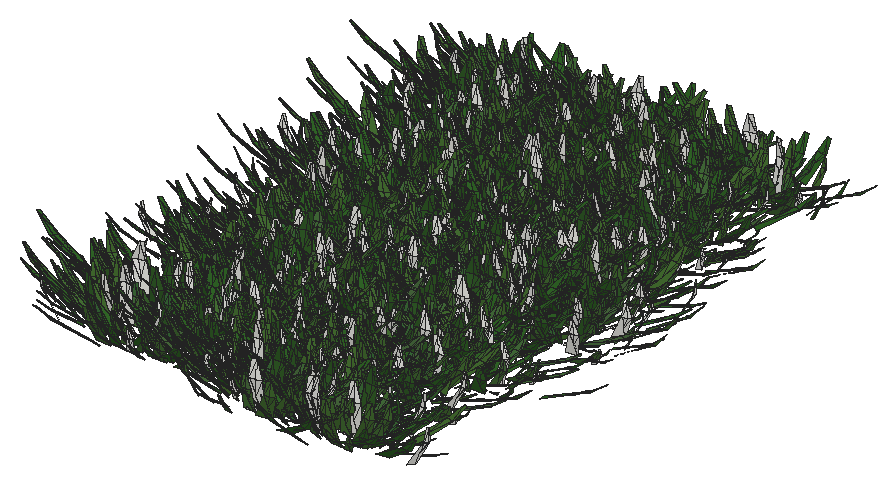
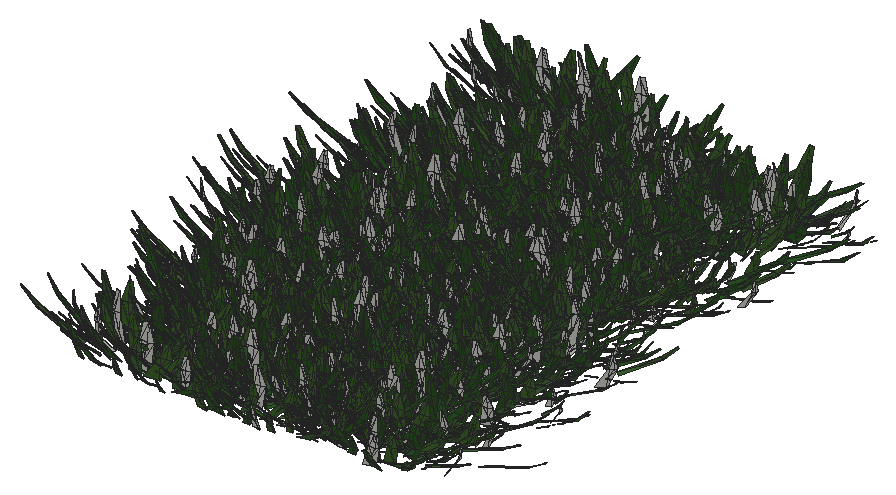
# SketchUp Ruby script. Lengths in inches.
U = 1.inch
M = Sketchup.active_model
def pt(a) = Geom::Point3d.new(a.map { |v| v * U })
def face(e, loops, mat)
  f = e.add_face(loops[0].map { |a| pt(a) })
  loops[1..].each { |l| e.add_face(l.map { |a| pt(a) }).erase! }
  f.material = f.back_material = mat if mat
  f
end
# faces: each face lists its corners as indices into pts; further lists are holes
def faces(e, pts, list, mat = nil) = list.each { |f| face(e, (f[0].is_a?(Array) ? f : [f]).map { |l| l.map { |i| pts[i] } }, mat) }
# xy, xz, yz: faces in a plane at the given z, y or x. An outline is a flat list of corners, or four numbers for a rectangle; further outlines are holes
def ring(l) = l.size == 4 ? [[l[0], l[1]], [l[2], l[1]], [l[2], l[3]], [l[0], l[3]]] : l.each_slice(2).to_a
def flat(e, list, mat, &to3) = list.each { |f| face(e, (f[0].is_a?(Array) ? f : [f]).map { |l| ring(l).map { |u, v| to3.(u, v) } }, mat) }
def xy(e, z, list, mat = nil) = flat(e, list, mat) { |x, y| [x, y, z] }
def xz(e, y, list, mat = nil) = flat(e, list, mat) { |x, z| [x, y, z] }
def yz(e, x, list, mat = nil) = flat(e, list, mat) { |y, z| [x, y, z] }
def lines(e, pts, list) = list.each { |a, b| e.add_line(pt(pts[a]), pt(pts[b])) }
# prism: a flat outline (further loops are holes) pulled along v
def prism(e, loops, v, mat = nil)
  f = face(e, loops, mat); d = Geom::Vector3d.new(v.map { |x| x * U })
  f.pushpull(f.normal.samedirection?(d) ? d.length : -d.length)
end
def box(e, o, s, mat = nil) = prism(e, [[o, [o[0] + s[0], o[1], o[2]], [o[0] + s[0], o[1] + s[1], o[2]], [o[0], o[1] + s[1], o[2]]]], [0, 0, s[2]], mat)
def at(x, y, z, deg = 0) = Geom::Transformation.translation(pt([x, y, z])) * Geom::Transformation.rotation(ORIGIN, Z_AXIS, deg.degrees)
def axes(o, x, y, z) = Geom::Transformation.new([*x, 0, *y, 0, *z, 0, *pt(o).to_a, 1])
def part(name) = M.definitions.add(name)
# library, detail: a bought-in or finely detailed component or shape, given as its bounding box
def library(name, o, s) = part(name).tap { |d| box(d.entities, o, s) }
def detail(e, o, s) = box(e.add_group.entities, o, s)
def put(e, d, t, mat = nil) = e.add_instance(d, t).tap { |i| i.material = mat if mat }
def group(e, t, mat = nil) = e.add_group.tap { |g| g.transformation = t; g.material = mat if mat }.entities
root = M.entities
M.materials.add("Material82").color = [68, 110, 58]
M.materials.add("Material83").color = [48, 90, 38]
M.materials.add("Material84").color = [68, 110, 48]
M.materials.add("Material85").color = [48, 90, 48]
M.materials.add("Material86").color = [58, 110, 58]
M.materials.add("Material87").color = [58, 90, 38]
M.materials.add("Material88").color = [68, 100, 58]
M.materials.add("Material89").color = [48, 100, 38]
c1 = part("grass00")
p = [[-0.6875,0.15,0],[-0.56,0.08,5.52],[-0.04,0.03,2.76],[0.48,-0.02,0],[0.35,-0.02,5.52],[-0.1,-0.14,5.52],
  [-0.12,0.65,8.37],[-0.42,0.65,8.37]]
faces(c1.entities,p,[[0,1,2,3],[3,2,4],[1,5,2],[5,4,2],[1,6,5],[4,5,6],[7,6,1]])
c2 = part("Group16\#1")
put(c2.entities,c1,axes([1.44,-0.61,-0.01],[0.05352,0.12609,0],[-0.10704,0.04543,0.07239],[0.06664,-0.02828,0.11628]),"Material85")
put(c2.entities,c1,axes([0.76,-0.15,-0.01],[0.04676,0.24062,0],[-0.23162,0.04501,0.06642],[0.0652,-0.01267,0.23595]),"Material82")
put(c2.entities,c1,axes([0.79,0.01,-0.01],[-0.00606,0.34651,0],[-0.34381,-0.00602,0.0432],[0.04319,0.00076,0.34386]))
put(c2.entities,c1,axes([1,0.23,-0.01],[-0.07192,0.31144,0],[-0.28722,-0.06632,0.1236],[0.12043,0.02781,0.29478]),"Material84")
put(c2.entities,c1,axes([1.66,0.77,-0.01],[-0.13828,0.29651,0],[-0.21551,-0.1005,0.22471],[0.20365,0.09498,0.23779]),"Material89")
put(c2.entities,c1,axes([0.6875,0.52,-0.01],[-0.18126,0.24051,0],[-0.22746,-0.17142,0.09788],[0.07817,0.05891,0.28481]),"Material84")
put(c2.entities,c1,axes([0.68,0.78,-0.01],[-0.215,0.18688,0],[-0.12385,-0.14248,0.21334],[0.13995,0.16101,0.18878]),"Material82")
put(c2.entities,c1,axes([0.56,1,-0.01],[-0.13756,0.07624,0],[-0.06159,-0.11112,0.0927],[0.04494,0.08108,0.12705]),"Material84")
put(c2.entities,c1,axes([0.2,0.64,-0.01],[-0.23729,0.07254,0],[-0.05711,-0.18681,0.153],[0.04473,0.14632,0.19535]),"Material89")
put(c2.entities,c1,axes([0.0625,0.72,-0.01],[-0.28874,0.02525,0],[-0.02179,-0.24916,0.14647],[0.01276,0.14591,0.25012]),"Material82")
put(c2.entities,c1,axes([-0.08,0.62,-0.01],[-0.34089,-0.04187,0],[0.03255,-0.26504,0.216],[-0.02633,0.21439,0.26703]),"Material89")
put(c2.entities,c1,axes([-0.34,0.98,-0.01],[-0.14314,-0.0493,0],[0.04397,-0.12769,0.06843],[-0.02228,0.0647,0.13505]),"Material89")
put(c2.entities,c1,axes([-0.87,1.45,-0.01],[-0.23488,-0.14114,0],[0.13761,-0.22901,0.06087],[-0.03135,0.05217,0.26717]))
put(c2.entities,c1,axes([-0.72,0.77,-0.01],[-0.14208,-0.13251,0],[0.07209,-0.0773,0.16301],[-0.11118,0.11922,0.1057]),"Material89")
put(c2.entities,c1,axes([-0.62,0.43,-0.01],[-0.14845,-0.21203,0],[0.18654,-0.13061,0.12304],[-0.10079,0.07057,0.22772]),"Material82")
put(c2.entities,c1,axes([-0.68,0.29,-0.01],[-0.13639,-0.32136,0],[0.31723,-0.13464,0.05579],[-0.05136,0.0218,0.34462]),"Material83")
put(c2.entities,c1,axes([-0.64,0.125,-0.01],[-0.0458,-0.23569,0],[0.22124,-0.043,0.08276],[-0.08124,0.01579,0.22538]),"Material86")
put(c2.entities,c1,axes([-1.6,-0.03,-0.01],[0.00576,-0.32897,0],[0.27526,0.00482,0.18018],[-0.18015,-0.00315,0.2753]),"Material84")
put(c2.entities,c1,axes([-1.36,-0.31,-0.01],[0.05718,-0.24765,0],[0.18172,0.04196,0.17267],[-0.16825,-0.03885,0.1865]),"Material89")
put(c2.entities,c1,axes([-1.54,-0.72,-0.01],[0.06537,-0.14017,0],[0.13555,0.06321,0.03939],[-0.0357,-0.01665,0.14956]))
put(c2.entities,c1,axes([-1.19,-0.9,-0.01],[0.09597,-0.12735,0],[0.11214,0.08451,0.07557],[-0.06035,-0.04548,0.14042]),"Material88")
put(c2.entities,c1,axes([-0.47,-0.54,-0.01],[0.11588,-0.10072,0],[0.0618,0.0711,0.12124],[-0.07953,-0.0915,0.0942]))
put(c2.entities,c1,axes([-0.47,-0.84,-0.01],[0.11927,-0.0661,0],[0.06603,0.11913,0.00646],[-0.00313,-0.00565,0.13621]),"Material84")
put(c2.entities,c1,axes([-0.38,-1.24,-0.01],[0.28037,-0.08571,0],[0.0618,0.20215,0.20315],[-0.05939,-0.19428,0.21139]),"Material88")
put(c2.entities,c1,axes([-0.06,-0.66,-0.01],[0.22719,-0.01987,0],[0.01247,0.14255,0.17758],[-0.01547,-0.17691,0.1431]),"Material87")
put(c2.entities,c1,axes([0.11,-0.89,-0.01],[0.14882,0.01828,0],[-0.01058,0.08611,0.12229],[0.01491,-0.12138,0.08676]),"Material85")
put(c2.entities,c1,axes([0.25,-0.72,-0.01],[0.20481,0.07053,0],[-0.06206,0.18022,0.10291],[0.03351,-0.0973,0.1906]),"Material85")
put(c2.entities,c1,axes([0.85,-1.42,-0.01],[0.16481,0.09904,0],[-0.09472,0.15762,0.05616],[0.02893,-0.04814,0.18389]),"Material84")
put(c2.entities,c1,axes([1.01,-1.09,-0.01],[0.21858,0.20385,0],[-0.17495,0.1876,0.15339],[0.10462,-0.11218,0.25652]),"Material89")
put(c2.entities,c1,axes([1.01,-0.71,-0.01],[0.08733,0.12473,0],[-0.06445,0.04512,0.13037],[0.1068,-0.07477,0.07867]),"Material85")
c3 = part("Group15\#1")
put(c3.entities,c2,at(0,0,0))
c4 = part("3darcstudiotree_grass00\#1")
put(c4.entities,c3,at(0,0,0))
put(root,c4,axes([656.28,960.15,-29.74],[-3.29694,-0.59268,0],[1.38855,-1.20133,-0.0331],[0.08455,-0.07315,1.54531]))
put(root,c4,axes([655.14,956.93,-29.74],[2.67683,1.25305,0],[-2.64635,0.87925,-0.04423],[-0.18001,0.05981,1.38013]))
put(root,c4,axes([656.28,979.83,-29.74],[1.85229,-1.14191,0],[3.43107,0.86561,-0.02581],[0.11483,0.02897,1.61243]))
put(root,c4,axes([656.78,970.66,-29.74],[-0.72323,-1.62263,0],[3.80365,-0.26368,-0.04893],[0.28769,-0.01994,1.72817]))
put(root,c4,axes([656.52,992.4,-29.74],[-3.72731,0.81099,0],[-1.84954,-1.32207,-0.01481],[-0.0358,-0.02559,1.43556]))
put(root,c4,axes([655.86,984.05,-29.74],[4.17155,-0.17702,0],[0.50263,1.84221,-0.03237],[0.01504,0.05512,1.52951]))
put(root,c4,axes([657.4,951.16,-29.74],[-4.25916,-0.67423,0],[1.26133,-1.23925,-0.04034],[0.09396,-0.09232,1.58691]))
put(root,c4,axes([657.34,976.97,-29.74],[-0.75362,-1.53541,0],[3.24661,-0.24784,-0.00678],[0.04146,-0.00316,1.54322]))
put(root,c4,axes([657.8,973.3,-29.74],[-2.20792,-1.57829,0],[3.78019,-0.82247,-0.0117],[0.05427,-0.01181,1.7149]))
put(root,c4,axes([656.19,996.11,-29.74],[1.20267,1.27774,0],[-3.21983,0.47135,-0.04291],[-0.22552,0.03301,1.44315]))
put(root,c4,axes([656.97,988.91,-29.74],[2.6006,-1.2072,0],[3.21281,1.07644,-0.02612],[0.11842,0.03968,1.8801]))
put(root,c4,axes([656.41,942.99,-29.74],[-0.33098,1.70392,0],[-3.92143,-0.11847,-0.03234],[-0.20787,-0.00628,1.90052]))
put(root,c4,axes([656.09,974.61,-29.74],[3.87339,1.05779,0],[-2.14052,1.21905,-0.05103],[-0.17397,0.09908,1.6877]))
put(root,c4,axes([656.49,943.82,-29.74],[4.23456,-0.44217,0],[1.03247,1.53783,-0.03329],[0.03822,0.05692,1.35616]))
put(root,c4,axes([657.375,947.27,-29.74],[-3.02099,1.21639,0],[-3.37871,-1.30508,-0.0181],[-0.07062,-0.02728,1.93624]))
put(root,c4,axes([658.08,962.33,-29.74],[1.13928,-1.32787,0],[4.00016,0.53378,-0.02846],[0.11467,0.0153,1.34635]))
put(root,c4,axes([658.56,964.12,-29.74],[1.43898,-1.34623,0],[3.17438,0.52772,-0.03331],[0.18037,0.02999,1.51731]))
put(root,c4,axes([658.57,985.71,-29.74],[-2.26233,1.10327,0],[-2.6855,-0.85647,-0.00747],[-0.03039,-0.00969,1.35493]))
put(root,c4,axes([658.69,990.84,-29.74],[0.61227,1.37165,0],[-4.42146,0.30696,-0.06022],[-0.31422,0.02181,1.78296]))
put(root,c4,axes([658.71,965.45,-29.74],[1.96702,1.06284,0],[-3.17968,0.91525,-0.05552],[-0.21201,0.06102,1.39481]))
put(root,c4,axes([660.65,995.01,-29.74],[-1.36397,-1.5291,0],[3.40561,-0.47247,-0.03242],[0.15123,-0.02098,1.33794]))
put(root,c4,axes([661.85,941.96,-29.74],[-3.87962,-0.67736,0],[1.4284,-1.27243,-0.0129],[0.02606,-0.02321,1.31952]))
put(root,c4,axes([660.875,980.75,-29.74],[-2.78639,1.08314,0],[-3.04744,-1.21928,-0.00446],[-0.01393,-0.00557,1.44777]))
put(root,c4,axes([661.83,967.76,-29.74],[-4.49573,0.21611,0],[-0.44378,-1.43584,-0.03065],[-0.02667,-0.0863,1.97713]))
put(root,c4,axes([662.33,991.92,-29.74],[-1.74555,-1.44076,0],[3.95857,-0.74592,-0.00689],[0.03295,-0.00621,1.74288]))
put(root,c4,axes([662.27,987.44,-29.74],[-3.15245,-0.45856,0],[1.56973,-1.67838,-0.02933],[0.05139,-0.05494,1.72129]))
put(root,c4,axes([661,996.1875,-29.74],[4.34464,0.20061,0],[-0.52956,1.78372,-0.02723],[-0.01491,0.05022,1.60719]))
put(root,c4,axes([661.39,946.51,-29.74],[3.87508,-0.19158,0],[0.55593,1.74888,-0.03701],[0.02742,0.08626,1.99511]))
put(root,c4,axes([661.15,973.63,-29.74],[4.00255,0.79486,0],[-1.95042,1.52752,-0.03278],[-0.08544,0.06692,1.8841]))
put(root,c4,axes([662.47,966.61,-29.74],[1.64847,-1.35078,0],[4.23243,0.80334,-0.06017],[0.26789,0.05085,1.73941]))
put(root,c4,axes([662.32,957.09,-29.74],[2.33049,-1.15129,0],[2.65609,0.83622,-0.01018],[0.04728,0.01488,1.51436]))
put(root,c4,axes([661.5625,983.62,-29.74],[3.64852,0.24315,0],[-0.61045,1.42466,-0.04218],[-0.04748,0.11082,1.85529]))
put(root,c4,axes([663.05,952.86,-29.74],[-1.10259,-1.32087,0],[4.19794,-0.54501,-0.05688],[0.29749,-0.03862,1.82396]))
put(root,c4,axes([661.5,962.37,-29.74],[4.20126,0.39077,0],[-0.91213,1.52518,-0.02883],[-0.04091,0.06841,1.84132]))
put(root,c4,axes([662.49,951.28,-29.74],[2.88399,-0.92183,0],[2.75264,1.33938,-0.02341],[0.07157,0.03482,1.59067]))
put(root,c4,axes([663.5625,974.9,-29.74],[-3.28835,-0.7389,0],[1.7462,-1.20864,-0.01205],[0.03007,-0.02081,1.33255]))
put(root,c4,axes([663.67,955.34,-29.74],[-3.05685,-0.82947,0],[2.14696,-1.23058,-0.02104],[0.07287,-0.04177,1.73448]))
put(root,c4,axes([663.6875,985.56,-29.74],[-2.64127,-0.90818,0],[2.55598,-1.15614,-0.03875],[0.14904,-0.06742,1.70607]))
put(root,c4,axes([662.95,959.7,-29.74],[2.49775,-0.87161,0],[2.87959,1.28342,-0.04815],[0.19249,0.08579,1.9649]))
put(root,c4,axes([662.71,989.8,-29.74],[3.57061,0.64267,0],[-1.40632,1.21522,-0.03533],[-0.10777,0.09312,1.86502]))
put(root,c4,axes([663.55,970.9375,-29.74],[3.75674,0.29184,0],[-0.86575,1.73332,-0.03192],[-0.02673,0.05352,1.45488]))
put(root,c4,axes([663.91,978.89,-29.74],[-0.44896,1.44211,0],[-4.03082,-0.19517,-0.03564],[-0.19872,-0.00962,1.71014]))
put(root,c4,axes([663.55,948.04,-29.74],[4.11072,0.52115,0],[-1.12592,1.38127,-0.00634],[-0.01225,0.01503,1.74238]))
put(root,c4,axes([664.4375,963.79,-29.74],[3.24027,-0.98547,0],[2.31887,1.18584,-0.00737],[0.02262,0.01157,1.42978]))
put(root,c4,axes([663.79,943.9,-29.74],[0.47172,1.49628,0],[-3.52699,0.17294,-0.00588],[-0.02991,0.00147,1.36568]))
put(root,c4,axes([663.7,977.6,-29.74],[2.55644,1.08061,0],[-3.46336,1.27432,-0.03325],[-0.10953,0.0403,1.59934]))
put(root,c4,axes([666,994.85,-29.74],[-3.55761,-0.37183,0],[0.9234,-1.37408,-0.01321],[0.02436,-0.03625,1.9444]))
put(root,c4,axes([666.29,962.64,-29.74],[-1.58706,-1.22315,0],[3.88697,-0.78439,-0.02541],[0.09132,-0.01843,1.32108]))
put(root,c4,axes([666.1,979.85,-29.74],[0.37581,-1.33084,0],[4.05324,0.17801,-0.00391],[0.01773,0.00078,1.39627]))
put(root,c4,axes([665.89,973.54,-29.74],[0.29138,-1.80133,0],[3.99838,0.10059,-0.05413],[0.25015,0.00629,1.39055]))
put(root,c4,axes([666.08,959.01,-29.74],[0.60335,-1.83981,0],[4.64218,0.23677,-0.05291],[0.19949,0.01017,1.33374]))
put(root,c4,axes([666.33,951.6,-29.74],[-4.16919,-0.21002,0],[0.49933,-1.5417,-0.0157],[0.01299,-0.04011,1.92971]))
put(root,c4,axes([666.4,992.99,-29.74],[0.3233,-1.61244,0],[3.70268,0.11546,-0.00365],[0.02017,0.00063,1.54435]))
put(root,c4,axes([666.46,970.72,-29.74],[2.70248,-1.34249,0],[3.67105,1.14936,-0.06314],[0.18316,0.05735,1.30132]))
put(root,c4,axes([666.62,949.09,-29.74],[-3.51608,0.58555,0],[-1.76508,-1.64843,-0.01449],[-0.02729,-0.02549,1.64714]))
put(root,c4,axes([667.89,996.89,-29.74],[-1.97159,-1.316,0],[4.00038,-0.93213,-0.05519],[0.24758,-0.05769,1.81465]))
put(root,c4,axes([666.03,964.21,-29.74],[2.05839,1.31648,0],[-3.03228,0.73739,-0.00763],[-0.03853,0.00937,1.58363]))
put(root,c4,axes([666.4375,976.98,-29.74],[3.97377,-0.0043,0],[0.0116,1.66593,-0.02008],[0.00028,0.04042,1.61638]))
put(root,c4,axes([666.5625,953.96,-29.74],[0.70204,1.43301,0],[-3.58325,0.27302,-0.03785],[-0.19362,0.01475,1.42505]))
put(root,c4,axes([668.22,989.69,-29.74],[-3.33443,-0.23634,0],[0.70723,-1.55188,-0.01818],[0.01451,-0.03184,1.35222]))
put(root,c4,axes([668.55,957.45,-29.74],[-4.02551,-0.90949,0],[2.09135,-1.43967,-0.04075],[0.0999,-0.06877,1.55523]))
put(root,c4,axes([666.69,975.52,-29.74],[4.20535,0.69684,0],[-1.48182,1.39084,-0.00848],[-0.02193,0.02058,1.91304]))
put(root,c4,axes([666.9,955.63,-29.74],[3.86131,0.54377,0],[-1.4335,1.58316,-0.00059],[-0.00108,0.0012,1.74794]))
put(root,c4,axes([668.26,983.61,-29.74],[2.33801,-1.27151,0],[3.45385,0.98774,-0.00976],[0.0468,0.01338,1.89325]))
put(root,c4,axes([668.59,985.51,-29.74],[-0.84806,-1.31842,0],[3.86352,-0.38651,-0.05601],[0.32758,-0.03277,1.80254]))
put(root,c4,axes([668.61,969.14,-29.74],[2.53276,-1.11904,0],[3.44801,1.21375,-0.02458],[0.09462,0.03331,1.78746]))
put(root,c4,axes([669.6,981.83,-29.74],[-3.79387,-0.48377,0],[1.38418,-1.6883,-0.04655],[0.0671,-0.08184,1.58019]))
put(root,c4,axes([668.33,946.28,-29.74],[3.58882,-0.43849,0],[1.01017,1.28588,-0.04073],[0.06773,0.08621,1.43775]))
put(root,c4,axes([668.37,944.61,-29.74],[1.5336,1.30723,0],[-4.13356,0.75421,-0.03574],[-0.18177,0.03317,1.91331]))
put(root,c4,axes([668.82,988.3125,-29.74],[4.25696,0.81021,0],[-1.71809,1.40397,-0.05424],[-0.1086,0.08874,1.36476]))
put(root,c4,axes([669.96,965.67,-29.74],[1.26993,-1.49927,0],[3.12751,0.41201,-0.03453],[0.23339,0.03075,1.76116]))
put(root,c4,axes([670.02,942.89,-29.74],[0.88446,1.28365,0],[-3.4154,0.366,-0.02204],[-0.14997,0.01607,1.87051]))
put(root,c4,axes([671.6,957.21,-29.74],[-4.2844,-0.03587,0],[0.08793,-1.63328,-0.04949],[0.00646,-0.12004,1.9102]))
put(root,c4,axes([672.58,986.64,-29.74],[-1.79663,-1.22383,0],[3.52148,-0.80403,-0.02105],[0.11606,-0.0265,1.94345]))
put(root,c4,axes([671.76,983.79,-29.74],[-3.1837,0.9292,0],[-2.49148,-1.32767,-0.01624],[-0.05606,-0.02987,1.82169]))
put(root,c4,axes([672.21,963.31,-29.74],[2.23016,-1.08828,0],[2.80047,0.89256,-0.01488],[0.0583,0.01858,1.35946]))
put(root,c4,axes([673.01,981.42,-29.74],[-2.22834,-1.37792,0],[3.47538,-0.87412,-0.04256],[0.18098,-0.04552,1.55835]))
put(root,c4,axes([671.78,992.89,-29.74],[3.33835,-0.04276,0],[0.15045,1.82678,-0.05593],[0.00839,0.10182,1.60461]))
put(root,c4,axes([673.13,989.77,-29.74],[0.7854,-1.46662,0],[3.6757,0.30614,-0.00249],[0.01359,0.00113,1.57305]))
put(root,c4,axes([672.46,996.89,-29.74],[-3.47223,1.22215,0],[-3.01377,-1.3317,-0.01139],[-0.0395,-0.01745,1.76647]))
put(root,c4,axes([673.61,995.18,-29.74],[-0.62966,-1.28695,0],[4.54348,-0.34574,-0.02161],[0.1197,-0.00911,1.95654]))
put(root,c4,axes([673.36,952.93,-29.74],[1.31559,-1.26739,0],[3.71813,0.60026,-0.00546],[0.02236,0.00361,1.33158]))
put(root,c4,axes([672.11,977.52,-29.74],[0.91997,1.29984,0],[-3.25818,0.35865,-0.02635],[-0.1448,0.01594,1.4463]))
put(root,c4,axes([672.54,987.94,-29.74],[-2.04292,1.4828,0],[-3.7482,-0.80316,-0.0267],[-0.09668,-0.02072,1.31753]))
put(root,c4,axes([673.6875,940.42,-29.74],[1.12764,-1.73077,0],[4.18377,0.42395,-0.01129],[0.06303,0.00639,1.86628]))
put(root,c4,axes([672.14,975.1875,-29.74],[3.72756,0.95688,0],[-1.9535,1.18357,-0.02904],[-0.10466,0.06341,1.7729]))
put(root,c4,axes([672.87,972.29,-29.74],[3.3945,-0.58791,0],[1.6844,1.5126,-0.00525],[0.01109,0.00996,1.64886]))
put(root,c4,axes([673.03,978.79,-29.74],[3.30024,-0.68967,0],[2.06464,1.53659,-0.00115],[0.00232,0.00173,1.42878]))
put(root,c4,axes([672.51,960.32,-29.74],[3.05854,0.58726,0],[-2.04234,1.65433,-0.05845],[-0.11264,0.09124,1.53958]))
put(root,c4,axes([674.18,950.68,-29.74],[-4.47684,0.54828,0],[-1.1065,-1.40519,-0.03919],[-0.07055,-0.08959,1.69748]))
put(root,c4,axes([673.05,968.63,-29.74],[4.02075,-0.11832,0],[0.27482,1.45248,-0.02534],[0.01078,0.05696,1.58232]))
put(root,c4,axes([673.61,945.09,-29.74],[3.57543,-0.38769,0],[0.94849,1.36047,-0.03828],[0.05948,0.08532,1.57185]))
put(root,c4,axes([673.44,971.41,-29.74],[3.70563,0.39578,0],[-0.96164,1.40032,-0.0432],[-0.06214,0.09049,1.51727]))
put(root,c4,axes([674.1875,947.01,-29.74],[-2.1552,1.3099,0],[-3.57978,-0.91604,-0.05659],[-0.20761,-0.05313,1.39892]))
put(root,c4,axes([675.27,966.39,-29.74],[2.80865,-0.79423,0],[2.35611,1.29587,-0.04704],[0.15431,0.08487,1.70604]))
put(root,c4,axes([674.46,942.25,-29.74],[3.02481,0.98705,0],[-2.84435,1.35567,-0.00662],[-0.02068,0.00986,1.63949]))
put(root,c4,axes([675.27,961.53,-29.74],[4.31211,0.22009,0],[-0.60247,1.83583,-0.04718],[-0.02535,0.07723,1.4726]))
put(root,c4,axes([675.54,948.86,-29.74],[0.84595,1.74988,0],[-3.45616,0.25986,-0.03349],[-0.2005,0.01508,1.60736]))
put(root,c4,axes([677.03,949.62,-29.74],[-2.74028,-0.81988,0],[2.08475,-1.08371,-0.01586],[0.05642,-0.02933,1.52204]))
put(root,c4,axes([675.5,955.56,-29.74],[3.77018,0.78532,0],[-1.755,1.3104,-0.05015],[-0.15166,0.11324,1.82381]))
put(root,c4,axes([677.04,969.24,-29.74],[3.19182,-1.13301,0],[2.43556,1.06713,-0.02235],[0.10598,0.04644,1.93391]))
put(root,c4,axes([677.67,975.73,-29.74],[2.31636,-1.46039,0],[3.68995,0.91026,-0.01393],[0.05236,0.01292,1.44657]))
put(root,c4,axes([677.72,995.14,-29.74],[-3.95397,0.70682,0],[-1.69994,-1.479,-0.00714],[-0.01245,-0.01084,1.30481]))
put(root,c4,axes([678,962.23,-29.74],[1.88589,-1.60822,0],[4.27567,0.77981,-0.01],[0.0511,0.00932,1.98774]))
put(root,c4,axes([677.22,960.27,-29.74],[-1.85089,1.19146,0],[-2.90652,-0.70224,-0.01687],[-0.07661,-0.01851,1.36079]))
put(root,c4,axes([678.46,941.74,-29.74],[1.40551,-1.64885,0],[4.26228,0.56508,-0.02131],[0.10181,0.0135,1.69918]))
put(root,c4,axes([677.82,955.81,-29.74],[2.41246,-1.41032,0],[3.04441,0.80995,-0.04469],[0.24595,0.06543,1.8275]))
put(root,c4,axes([677.74,997.6,-29.74],[-0.9909,1.30306,0],[-3.23471,-0.38257,-0.04553],[-0.22482,-0.02659,1.30482]))
put(root,c4,axes([678.92,973.16,-29.74],[-2.9141,-1.11595,0],[2.66035,-1.08046,-0.03796],[0.14613,-0.05935,1.58175]))
put(root,c4,axes([677.36,987.78,-29.74],[-0.05283,1.30539,0],[-4.56112,-0.02871,-0.04794],[-0.23084,-0.00145,1.64652]))
put(root,c4,axes([678.45,976.38,-29.74],[1.60686,-1.51832,0],[3.56667,0.58707,-0.05171],[0.27066,0.04455,1.64301]))
put(root,c4,axes([679.59,990.74,-29.74],[-1.63027,-1.73131,0],[4.11958,-0.60332,-0.00006],[0.00033,-0.00005,1.81412]))
put(root,c4,axes([677.96,992.01,-29.74],[0.46872,1.37145,0],[-4.27579,0.22728,-0.05207],[-0.28533,0.01517,1.7882]))
put(root,c4,axes([679.56,950.47,-29.74],[-3.00354,-1.31894,0],[3.37135,-1.19405,-0.05274],[0.22952,-0.08129,1.98669]))
put(root,c4,axes([677.92,944.83,-29.74],[0.98392,1.60393,0],[-4.31274,0.41147,-0.01063],[-0.04621,0.00441,1.48723]))
put(root,c4,axes([678.69,985.38,-29.74],[4.05845,0.38101,0],[-1.01694,1.68476,-0.06215],[-0.0714,0.11828,1.63292]))
put(root,c4,axes([680.51,979.07,-29.74],[-3.29654,-0.72222,0],[2.17338,-1.54289,-0.02959],[0.0707,-0.05019,1.65043]))
put(root,c4,axes([678.93,983.92,-29.74],[1.47468,1.38827,0],[-3.83437,0.63347,-0.03717],[-0.17802,0.02941,1.61797]))
put(root,c4,axes([678.94,964.12,-29.74],[2.9165,0.98147,0],[-2.52132,1.16527,-0.03219],[-0.13562,0.06268,1.88986]))
put(root,c4,axes([678.73,945.96,-29.74],[2.31946,1.24356,0],[-3.54601,1.02866,-0.02079],[-0.06877,0.01995,1.35493]))
put(root,c4,axes([680.9375,981.77,-29.74],[-4.41332,-0.66754,0],[1.63018,-1.67623,-0.02874],[0.04038,-0.04152,1.33872]))
put(root,c4,axes([680.41,971.08,-29.74],[-2.71187,1.03836,0],[-2.98144,-1.21104,-0.01854],[-0.0717,-0.02913,1.78092]))
put(root,c4,axes([680.38,957.99,-29.74],[4.10034,-0.52862,0],[1.2552,1.51427,-0.04269],[0.08479,0.10229,1.93529]))
put(root,c4,axes([680.99,953.07,-29.74],[2.75881,-1.06303,0],[3.05708,1.23394,-0.03867],[0.14354,0.05794,1.7417]))
put(root,c4,axes([680.61,966.5625,-29.74],[-0.60337,1.5081,0],[-3.83662,-0.23874,-0.0149],[-0.0971,-0.00604,1.9212]))
put(root,c4,axes([682.97,972.65,-29.74],[-3.93883,-1.01936,0],[1.86002,-1.11781,-0.04657],[0.18505,-0.11121,1.84036]))
put(root,c4,axes([682.68,942.04,-29.74],[1.31732,-1.5277,0],[3.94533,0.52911,-0.01889],[0.1126,0.0151,1.96679]))
put(root,c4,axes([682.58,979.33,-29.74],[2.55399,-1.11237,0],[2.83561,1.01258,-0.04299],[0.17745,0.06336,1.59659]))
put(root,c4,axes([683.48,940.71,-29.74],[-3.03372,-1.40875,0],[3.08967,-1.03482,-0.05304],[0.26,-0.08708,1.95407]))
put(root,c4,axes([683.42,981.73,-29.74],[-4.27576,-0.00967,0],[0.01971,-1.35519,-0.00073],[0.00002,-0.00168,1.50826]))
put(root,c4,axes([682.78,983.67,-29.74],[-2.10798,1.40451,0],[-3.51427,-0.82033,-0.03668],[-0.20421,-0.04767,1.98009]))
put(root,c4,axes([683.18,958.95,-29.74],[-3.10894,1.29688,0],[-2.64938,-0.9878,-0.02847],[-0.10631,-0.03964,1.40417]))
put(root,c4,axes([683.62,985.5,-29.74],[-3.43779,0.5694,0],[-1.45981,-1.37078,-0.01995],[-0.04437,-0.04166,1.62326]))
put(root,c4,axes([683.01,997.06,-29.74],[-1.73682,1.47733,0],[-4.1333,-0.75577,-0.04346],[-0.21523,-0.03935,1.86413]))
put(root,c4,axes([683.28,949.3125,-29.74],[-2.48253,1.23787,0],[-2.67891,-0.83558,-0.01059],[-0.04346,-0.01356,1.33934]))
put(root,c4,axes([684.23,968.86,-29.74],[-4.54038,0.15264,0],[-0.30495,-1.41082,-0.04632],[-0.02774,-0.12834,1.89764]))
put(root,c4,axes([682.64,988.71,-29.74],[3.62862,0.35052,0],[-1.11939,1.8023,-0.01455],[-0.01942,0.03128,1.97892]))
put(root,c4,axes([685.16,969.85,-29.74],[-4.13743,-0.67569,0],[1.3247,-1.26157,-0.00358],[0.00873,-0.00832,1.65637]))
put(root,c4,axes([684.25,976.7,-29.74],[-1.22945,1.37189,0],[-3.12548,-0.43563,-0.03966],[-0.20868,-0.02909,1.38647]))
put(root,c4,axes([684.73,964.71,-29.74],[-3.50072,1.23157,0],[-2.52643,-1.11691,-0.04505],[-0.14682,-0.06491,1.39266]))
put(root,c4,axes([685.67,974.22,-29.74],[-1.35898,-1.3893,0],[3.82798,-0.58237,-0.03571],[0.20852,-0.03172,1.92492]))
put(root,c4,axes([684.27,994.8,-29.74],[1.95907,1.41788,0],[-3.34699,0.71925,-0.025],[-0.15312,0.03291,1.99255]))
put(root,c4,axes([685.92,966.24,-29.74],[-4.10859,0.05118,0],[-0.12582,-1.57107,-0.03959],[-0.00691,-0.08629,1.65212]))
put(root,c4,axes([685.0625,955.9,-29.74],[3.60532,-0.46019,0],[1.33734,1.62954,-0.01611],[0.02411,0.02937,1.58139]))
